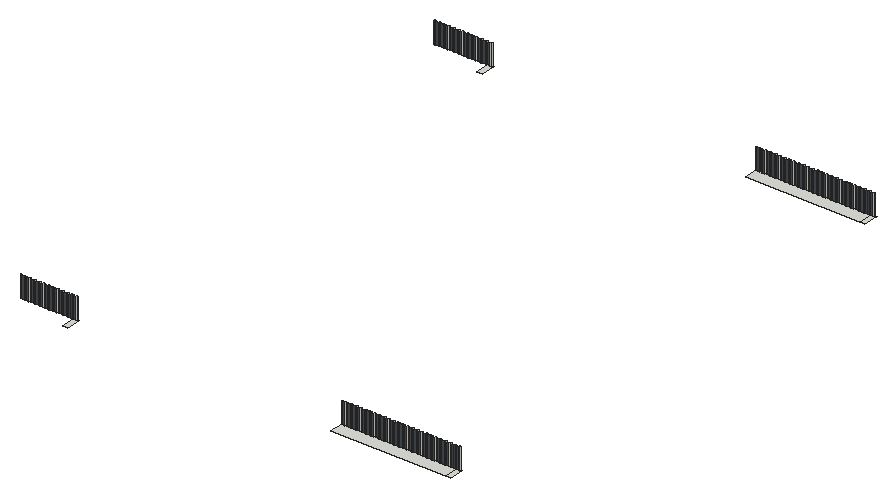
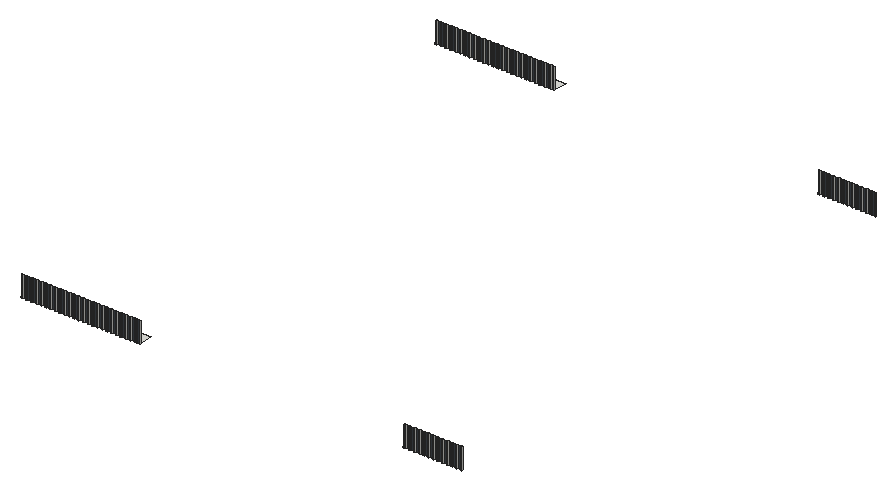
# SketchUp Ruby script. Lengths in inches.
U = 1.inch
M = Sketchup.active_model
def pt(a) = Geom::Point3d.new(a.map { |v| v * U })
def face(e, loops, mat)
  f = e.add_face(loops[0].map { |a| pt(a) })
  loops[1..].each { |l| e.add_face(l.map { |a| pt(a) }).erase! }
  f.material = f.back_material = mat if mat
  f
end
# faces: each face lists its corners as indices into pts; further lists are holes
def faces(e, pts, list, mat = nil) = list.each { |f| face(e, (f[0].is_a?(Array) ? f : [f]).map { |l| l.map { |i| pts[i] } }, mat) }
# xy, xz, yz: faces in a plane at the given z, y or x. An outline is a flat list of corners, or four numbers for a rectangle; further outlines are holes
def ring(l) = l.size == 4 ? [[l[0], l[1]], [l[2], l[1]], [l[2], l[3]], [l[0], l[3]]] : l.each_slice(2).to_a
def flat(e, list, mat, &to3) = list.each { |f| face(e, (f[0].is_a?(Array) ? f : [f]).map { |l| ring(l).map { |u, v| to3.(u, v) } }, mat) }
def xy(e, z, list, mat = nil) = flat(e, list, mat) { |x, y| [x, y, z] }
def xz(e, y, list, mat = nil) = flat(e, list, mat) { |x, z| [x, y, z] }
def yz(e, x, list, mat = nil) = flat(e, list, mat) { |y, z| [x, y, z] }
def lines(e, pts, list) = list.each { |a, b| e.add_line(pt(pts[a]), pt(pts[b])) }
# prism: a flat outline (further loops are holes) pulled along v
def prism(e, loops, v, mat = nil)
  f = face(e, loops, mat); d = Geom::Vector3d.new(v.map { |x| x * U })
  f.pushpull(f.normal.samedirection?(d) ? d.length : -d.length)
end
def box(e, o, s, mat = nil) = prism(e, [[o, [o[0] + s[0], o[1], o[2]], [o[0] + s[0], o[1] + s[1], o[2]], [o[0], o[1] + s[1], o[2]]]], [0, 0, s[2]], mat)
def at(x, y, z, deg = 0) = Geom::Transformation.translation(pt([x, y, z])) * Geom::Transformation.rotation(ORIGIN, Z_AXIS, deg.degrees)
def axes(o, x, y, z) = Geom::Transformation.new([*x, 0, *y, 0, *z, 0, *pt(o).to_a, 1])
def part(name) = M.definitions.add(name)
# library, detail: a bought-in or finely detailed component or shape, given as its bounding box
def library(name, o, s) = part(name).tap { |d| box(d.entities, o, s) }
def detail(e, o, s) = box(e.add_group.entities, o, s)
def put(e, d, t, mat = nil) = e.add_instance(d, t).tap { |i| i.material = mat if mat }
def group(e, t, mat = nil) = e.add_group.tap { |g| g.transformation = t; g.material = mat if mat }.entities
root = M.entities
M.materials.add("[Formica Blue]").color = [73, 80, 86]
xy(root,693.65,[[1078.41,412.04,1088.17,412.04,1088.17,437.1,1085.74,437.1,1085.74,438.72,1083.18,438.72,1083.18,437.1,1078.41,437.1],[1586.375,412.04,1802.84,412.04,1802.84,437.1,1801.29,437.1,1801.29,438.72,1798.73,438.72,1798.73,437.1,1792.39,437.1,1792.39,438.72,1789.84,438.72,1789.84,437.1,1783.5,437.1,1783.5,438.72,1780.95,438.72,1780.95,437.1,1774.61,437.1,1774.61,438.72,1772.05,438.72,1772.05,437.1,1765.72,437.1,1765.72,438.72,1763.16,438.72,1763.16,437.1,1756.83,437.1,1756.83,438.72,1754.27,438.72,1754.27,437.1,1747.9375,437.1,1747.9375,438.72,1745.38,438.72,1745.38,437.1,1739.05,437.1,1739.05,438.72,1736.49,438.72,1736.49,437.1,1730.16,437.1,1730.16,438.72,1727.6,438.72,1727.6,437.1,1721.26,437.1,1721.26,438.72,1718.71,438.72,1718.71,437.1,1712.375,437.1,1712.375,438.72,1709.82,438.72,1709.82,437.1,1703.48,437.1,1703.48,438.72,1700.92,438.72,1700.92,437.1,1694.59,437.1,1694.59,438.72,1692.03,438.72,1692.03,437.1,1685.7,437.1,1685.7,438.72,1683.14,438.72,1683.14,437.1,1676.81,437.1,1676.81,438.72,1674.25,438.72,1674.25,437.1,1667.92,437.1,1667.92,438.72,1665.36,438.72,1665.36,437.1,1659.03,437.1,1659.03,438.72,1656.47,438.72,1656.47,437.1,1650.13,437.1,1650.13,438.72,1647.58,438.72,1647.58,437.1,1641.24,437.1,1641.24,438.72,1638.69,438.72,1638.69,437.1,1632.35,437.1,1632.35,438.72,1629.79,438.72,1629.79,437.1,1623.46,437.1,1623.46,438.72,1620.9,438.72,1620.9,437.1,1614.57,437.1,1614.57,438.72,1612.01,438.72,1612.01,437.1,1605.68,437.1,1605.68,438.72,1603.12,438.72,1603.12,437.1,1596.79,437.1,1596.79,438.72,1592.81,438.72,1592.81,437.1,1586.47,437.1,1586.47,438.72,1586.375,438.72],[1802.84,412.04,1812.6,412.04,1812.6,437.1,1810.18,437.1,1810.18,438.72,1807.62,438.72,1807.62,437.1,1802.84,437.1],[1085.74,437.1,1088.17,438.72],[1810.18,437.1,1812.6,438.72],
  [1078.41,1392.39,1088.17,1392.39,1088.17,1417.45,1085.74,1417.45,1085.74,1419.07,1083.18,1419.07,1083.18,1417.45,1078.41,1417.45],[1586.375,1392.39,1802.84,1392.39,1802.84,1417.45,1801.29,1417.45,1801.29,1419.07,1798.73,1419.07,1798.73,1417.45,1792.39,1417.45,1792.39,1419.07,1789.84,1419.07,1789.84,1417.45,1783.5,1417.45,1783.5,1419.07,1780.95,1419.07,1780.95,1417.45,1774.61,1417.45,1774.61,1419.07,1772.05,1419.07,1772.05,1417.45,1765.72,1417.45,1765.72,1419.07,1763.16,1419.07,1763.16,1417.45,1756.83,1417.45,1756.83,1419.07,1754.27,1419.07,1754.27,1417.45,1747.9375,1417.45,1747.9375,1419.07,1745.38,1419.07,1745.38,1417.45,1739.05,1417.45,1739.05,1419.07,1736.49,1419.07,1736.49,1417.45,1730.16,1417.45,1730.16,1419.07,1727.6,1419.07,1727.6,1417.45,1721.26,1417.45,1721.26,1419.07,1718.71,1419.07,1718.71,1417.45,1712.375,1417.45,1712.375,1419.07,1709.82,1419.07,1709.82,1417.45,1703.48,1417.45,1703.48,1419.07,1700.92,1419.07,1700.92,1417.45,1694.59,1417.45,1694.59,1419.07,1692.03,1419.07,1692.03,1417.45,1685.7,1417.45,1685.7,1419.07,1683.14,1419.07,1683.14,1417.45,1676.81,1417.45,1676.81,1419.07,1674.25,1419.07,1674.25,1417.45,1667.92,1417.45,1667.92,1419.07,1665.36,1419.07,1665.36,1417.45,1659.03,1417.45,1659.03,1419.07,1656.47,1419.07,1656.47,1417.45,1650.13,1417.45,1650.13,1419.07,1647.58,1419.07,1647.58,1417.45,1641.24,1417.45,1641.24,1419.07,1638.69,1419.07,1638.69,1417.45,1632.35,1417.45,1632.35,1419.07,1629.79,1419.07,1629.79,1417.45,1623.46,1417.45,1623.46,1419.07,1620.9,1419.07,1620.9,1417.45,1614.57,1417.45,1614.57,1419.07,1612.01,1419.07,1612.01,1417.45,1605.68,1417.45,1605.68,1419.07,1603.12,1419.07,1603.12,1417.45,1596.79,1417.45,1596.79,1419.07,1592.81,1419.07,1592.81,1417.45,1586.47,1417.45,1586.47,1419.07,1586.375,1419.07],[1802.84,1392.39,1812.6,1392.39,1812.6,1417.45,1810.18,1417.45,1810.18,1419.07,1807.62,1419.07,1807.62,1417.45,1802.84,1417.45],[1085.74,1417.45,1088.17,1419.07],[1810.18,1417.45,1812.6,1419.07]])
xz(root,437.1,[[979.04,693.65,985.38,733.125],[987.9375,693.65,994.27,733.125],[996.83,693.65,1003.16,733.125],[1005.72,693.65,1012.05,733.125],[1014.61,693.65,1020.94,733.125],
  [1023.5,693.65,1029.83,733.125],[1032.39,693.65,1038.73,733.125],[1041.28,693.65,1047.62,733.125],[1050.17,693.65,1056.51,733.125],[1059.07,693.65,1065.4,733.125],
  [1067.96,693.65,1074.29,733.125],[1076.85,693.65,1083.18,733.125],[1586.47,693.65,1592.81,733.125],[1596.79,693.65,1603.12,733.125],[1605.68,693.65,1612.01,733.125],
  [1614.57,693.65,1620.9,733.125],[1623.46,693.65,1629.79,733.125],[1632.35,693.65,1638.69,733.125],[1641.24,693.65,1647.58,733.125],[1650.13,693.65,1656.47,733.125],
  [1659.03,693.65,1665.36,733.125],[1667.92,693.65,1674.25,733.125],[1676.81,693.65,1683.14,733.125],[1685.7,693.65,1692.03,733.125],[1694.59,693.65,1700.92,733.125],
  [1703.48,693.65,1709.82,733.125],[1712.375,693.65,1718.71,733.125],[1721.26,693.65,1727.6,733.125],[1730.16,693.65,1736.49,733.125],[1739.05,693.65,1745.38,733.125],
  [1747.9375,693.65,1754.27,733.125],[1756.83,693.65,1763.16,733.125],[1765.72,693.65,1772.05,733.125],[1774.61,693.65,1780.95,733.125],[1783.5,693.65,1789.84,733.125],
  [1792.39,693.65,1798.73,733.125],[1801.29,693.65,1807.62,733.125]],"[Formica Blue]")
xz(root,438.72,[[1586.375,693.65,1586.47,733.125]])
xz(root,438.72,[[976.49,693.65,979.04,733.125],[985.38,693.65,987.9375,733.125],[994.27,693.65,996.83,733.125],[1003.16,693.65,1005.72,733.125],[1012.05,693.65,1014.61,733.125],
  [1020.94,693.65,1023.5,733.125],[1029.83,693.65,1032.39,733.125],[1038.73,693.65,1041.28,733.125],[1047.62,693.65,1050.17,733.125],[1056.51,693.65,1059.07,733.125],
  [1065.4,693.65,1067.96,733.125],[1074.29,693.65,1076.85,733.125],[1083.18,693.65,1085.74,733.125],[1592.81,693.65,1596.79,733.125],[1603.12,693.65,1605.68,733.125],
  [1612.01,693.65,1614.57,733.125],[1620.9,693.65,1623.46,733.125],[1629.79,693.65,1632.35,733.125],[1638.69,693.65,1641.24,733.125],[1647.58,693.65,1650.13,733.125],
  [1656.47,693.65,1659.03,733.125],[1665.36,693.65,1667.92,733.125],[1674.25,693.65,1676.81,733.125],[1683.14,693.65,1685.7,733.125],[1692.03,693.65,1694.59,733.125],
  [1700.92,693.65,1703.48,733.125],[1709.82,693.65,1712.375,733.125],[1718.71,693.65,1721.26,733.125],[1727.6,693.65,1730.16,733.125],[1736.49,693.65,1739.05,733.125],
  [1745.38,693.65,1747.9375,733.125],[1754.27,693.65,1756.83,733.125],[1763.16,693.65,1765.72,733.125],[1772.05,693.65,1774.61,733.125],[1780.95,693.65,1783.5,733.125],
  [1789.84,693.65,1792.39,733.125],[1798.73,693.65,1801.29,733.125],[1807.62,693.65,1810.18,733.125]],"[Formica Blue]")
xz(root,1417.45,[[979.04,693.65,985.38,733.125],[987.9375,693.65,994.27,733.125],[996.83,693.65,1003.16,733.125],[1005.72,693.65,1012.05,733.125],[1014.61,693.65,1020.94,733.125],
  [1023.5,693.65,1029.83,733.125],[1032.39,693.65,1038.73,733.125],[1041.28,693.65,1047.62,733.125],[1050.17,693.65,1056.51,733.125],[1059.07,693.65,1065.4,733.125],
  [1067.96,693.65,1074.29,733.125],[1076.85,693.65,1083.18,733.125],[1586.47,693.65,1592.81,733.125],[1596.79,693.65,1603.12,733.125],[1605.68,693.65,1612.01,733.125],
  [1614.57,693.65,1620.9,733.125],[1623.46,693.65,1629.79,733.125],[1632.35,693.65,1638.69,733.125],[1641.24,693.65,1647.58,733.125],[1650.13,693.65,1656.47,733.125],
  [1659.03,693.65,1665.36,733.125],[1667.92,693.65,1674.25,733.125],[1676.81,693.65,1683.14,733.125],[1685.7,693.65,1692.03,733.125],[1694.59,693.65,1700.92,733.125],
  [1703.48,693.65,1709.82,733.125],[1712.375,693.65,1718.71,733.125],[1721.26,693.65,1727.6,733.125],[1730.16,693.65,1736.49,733.125],[1739.05,693.65,1745.38,733.125],
  [1747.9375,693.65,1754.27,733.125],[1756.83,693.65,1763.16,733.125],[1765.72,693.65,1772.05,733.125],[1774.61,693.65,1780.95,733.125],[1783.5,693.65,1789.84,733.125],
  [1792.39,693.65,1798.73,733.125],[1801.29,693.65,1807.62,733.125]],"[Formica Blue]")
xz(root,1419.07,[[1586.375,693.65,1586.47,733.125]])
xz(root,1419.07,[[976.49,693.65,979.04,733.125],[985.38,693.65,987.9375,733.125],[994.27,693.65,996.83,733.125],[1003.16,693.65,1005.72,733.125],[1012.05,693.65,1014.61,733.125],
  [1020.94,693.65,1023.5,733.125],[1029.83,693.65,1032.39,733.125],[1038.73,693.65,1041.28,733.125],[1047.62,693.65,1050.17,733.125],[1056.51,693.65,1059.07,733.125],
  [1065.4,693.65,1067.96,733.125],[1074.29,693.65,1076.85,733.125],[1083.18,693.65,1085.74,733.125],[1592.81,693.65,1596.79,733.125],[1603.12,693.65,1605.68,733.125],
  [1612.01,693.65,1614.57,733.125],[1620.9,693.65,1623.46,733.125],[1629.79,693.65,1632.35,733.125],[1638.69,693.65,1641.24,733.125],[1647.58,693.65,1650.13,733.125],
  [1656.47,693.65,1659.03,733.125],[1665.36,693.65,1667.92,733.125],[1674.25,693.65,1676.81,733.125],[1683.14,693.65,1685.7,733.125],[1692.03,693.65,1694.59,733.125],
  [1700.92,693.65,1703.48,733.125],[1709.82,693.65,1712.375,733.125],[1718.71,693.65,1721.26,733.125],[1727.6,693.65,1730.16,733.125],[1736.49,693.65,1739.05,733.125],
  [1745.38,693.65,1747.9375,733.125],[1754.27,693.65,1756.83,733.125],[1763.16,693.65,1765.72,733.125],[1772.05,693.65,1774.61,733.125],[1780.95,693.65,1783.5,733.125],
  [1789.84,693.65,1792.39,733.125],[1798.73,693.65,1801.29,733.125],[1807.62,693.65,1810.18,733.125]],"[Formica Blue]")
yz(root,976.49,[[1417.45,693.65,1419.07,733.125]])
yz(root,979.04,[[437.1,693.65,438.72,733.125],[1417.45,693.65,1419.07,733.125]])
yz(root,985.38,[[437.1,693.65,438.72,733.125],[1417.45,693.65,1419.07,733.125]])
yz(root,987.9375,[[437.1,693.65,438.72,733.125],[1417.45,693.65,1419.07,733.125]])
yz(root,994.27,[[437.1,693.65,438.72,733.125],[1417.45,693.65,1419.07,733.125]])
yz(root,996.83,[[437.1,693.65,438.72,733.125],[1417.45,693.65,1419.07,733.125]])
yz(root,1003.16,[[437.1,693.65,438.72,733.125],[1417.45,693.65,1419.07,733.125]])
yz(root,1005.72,[[437.1,693.65,438.72,733.125],[1417.45,693.65,1419.07,733.125]])
yz(root,1012.05,[[437.1,693.65,438.72,733.125],[1417.45,693.65,1419.07,733.125]])
yz(root,1014.61,[[437.1,693.65,438.72,733.125],[1417.45,693.65,1419.07,733.125]])
yz(root,1020.94,[[437.1,693.65,438.72,733.125],[1417.45,693.65,1419.07,733.125]])
yz(root,1023.5,[[437.1,693.65,438.72,733.125],[1417.45,693.65,1419.07,733.125]])
yz(root,1029.83,[[437.1,693.65,438.72,733.125],[1417.45,693.65,1419.07,733.125]])
yz(root,1032.39,[[437.1,693.65,438.72,733.125],[1417.45,693.65,1419.07,733.125]])
yz(root,1038.73,[[437.1,693.65,438.72,733.125],[1417.45,693.65,1419.07,733.125]])
yz(root,1041.28,[[437.1,693.65,438.72,733.125],[1417.45,693.65,1419.07,733.125]])
yz(root,1047.62,[[437.1,693.65,438.72,733.125],[1417.45,693.65,1419.07,733.125]])
yz(root,1050.17,[[437.1,693.65,438.72,733.125],[1417.45,693.65,1419.07,733.125]])
yz(root,1056.51,[[437.1,693.65,438.72,733.125],[1417.45,693.65,1419.07,733.125]])
yz(root,1059.07,[[437.1,693.65,438.72,733.125],[1417.45,693.65,1419.07,733.125]])
yz(root,1065.4,[[437.1,693.65,438.72,733.125],[1417.45,693.65,1419.07,733.125]])
yz(root,1067.96,[[437.1,693.65,438.72,733.125],[1417.45,693.65,1419.07,733.125]])
yz(root,1074.29,[[437.1,693.65,438.72,733.125],[1417.45,693.65,1419.07,733.125]],"[Formica Blue]")
yz(root,1076.85,[[437.1,693.65,438.72,733.125],[1417.45,693.65,1419.07,733.125]])
yz(root,1083.18,[[437.1,693.65,438.72,733.125],[1417.45,693.65,1419.07,733.125]])
yz(root,1085.74,[[437.1,693.65,438.72,733.125],[1417.45,693.65,1419.07,733.125]])
yz(root,1586.47,[[437.1,693.65,438.72,733.125],[1417.45,693.65,1419.07,733.125]])
yz(root,1592.81,[[437.1,693.65,438.72,733.125],[1417.45,693.65,1419.07,733.125]])
yz(root,1596.79,[[437.1,693.65,438.72,733.125],[1417.45,693.65,1419.07,733.125]])
yz(root,1603.12,[[437.1,693.65,438.72,733.125],[1417.45,693.65,1419.07,733.125]])
yz(root,1605.68,[[437.1,693.65,438.72,733.125],[1417.45,693.65,1419.07,733.125]])
yz(root,1612.01,[[437.1,693.65,438.72,733.125],[1417.45,693.65,1419.07,733.125]])
yz(root,1614.57,[[437.1,693.65,438.72,733.125],[1417.45,693.65,1419.07,733.125]])
yz(root,1620.9,[[437.1,693.65,438.72,733.125],[1417.45,693.65,1419.07,733.125]])
yz(root,1623.46,[[437.1,693.65,438.72,733.125],[1417.45,693.65,1419.07,733.125]])
yz(root,1629.79,[[437.1,693.65,438.72,733.125],[1417.45,693.65,1419.07,733.125]])
yz(root,1632.35,[[437.1,693.65,438.72,733.125],[1417.45,693.65,1419.07,733.125]])
yz(root,1638.69,[[437.1,693.65,438.72,733.125],[1417.45,693.65,1419.07,733.125]])
yz(root,1641.24,[[437.1,693.65,438.72,733.125],[1417.45,693.65,1419.07,733.125]])
yz(root,1647.58,[[437.1,693.65,438.72,733.125],[1417.45,693.65,1419.07,733.125]])
yz(root,1650.13,[[437.1,693.65,438.72,733.125],[1417.45,693.65,1419.07,733.125]])
yz(root,1656.47,[[437.1,693.65,438.72,733.125],[1417.45,693.65,1419.07,733.125]])
yz(root,1659.03,[[437.1,693.65,438.72,733.125],[1417.45,693.65,1419.07,733.125]])
yz(root,1665.36,[[437.1,693.65,438.72,733.125],[1417.45,693.65,1419.07,733.125]])
yz(root,1667.92,[[437.1,693.65,438.72,733.125],[1417.45,693.65,1419.07,733.125]])
yz(root,1674.25,[[437.1,693.65,438.72,733.125],[1417.45,693.65,1419.07,733.125]])
yz(root,1676.81,[[437.1,693.65,438.72,733.125],[1417.45,693.65,1419.07,733.125]])
yz(root,1683.14,[[437.1,693.65,438.72,733.125],[1417.45,693.65,1419.07,733.125]])
yz(root,1685.7,[[437.1,693.65,438.72,733.125],[1417.45,693.65,1419.07,733.125]])
yz(root,1692.03,[[437.1,693.65,438.72,733.125],[1417.45,693.65,1419.07,733.125]])
yz(root,1694.59,[[437.1,693.65,438.72,733.125],[1417.45,693.65,1419.07,733.125]])
yz(root,1700.92,[[437.1,693.65,438.72,733.125],[1417.45,693.65,1419.07,733.125]])
yz(root,1703.48,[[437.1,693.65,438.72,733.125],[1417.45,693.65,1419.07,733.125]])
yz(root,1709.82,[[437.1,693.65,438.72,733.125],[1417.45,693.65,1419.07,733.125]])
yz(root,1712.375,[[437.1,693.65,438.72,733.125],[1417.45,693.65,1419.07,733.125]])
yz(root,1718.71,[[437.1,693.65,438.72,733.125],[1417.45,693.65,1419.07,733.125]])
yz(root,1721.26,[[437.1,693.65,438.72,733.125],[1417.45,693.65,1419.07,733.125]])
yz(root,1727.6,[[437.1,693.65,438.72,733.125],[1417.45,693.65,1419.07,733.125]])
yz(root,1730.16,[[437.1,693.65,438.72,733.125],[1417.45,693.65,1419.07,733.125]])
yz(root,1736.49,[[437.1,693.65,438.72,733.125],[1417.45,693.65,1419.07,733.125]])
yz(root,1739.05,[[437.1,693.65,438.72,733.125],[1417.45,693.65,1419.07,733.125]])
yz(root,1745.38,[[437.1,693.65,438.72,733.125],[1417.45,693.65,1419.07,733.125]])
yz(root,1747.9375,[[437.1,693.65,438.72,733.125],[1417.45,693.65,1419.07,733.125]])
yz(root,1754.27,[[437.1,693.65,438.72,733.125],[1417.45,693.65,1419.07,733.125]])
yz(root,1756.83,[[437.1,693.65,438.72,733.125],[1417.45,693.65,1419.07,733.125]])
yz(root,1763.16,[[437.1,693.65,438.72,733.125],[1417.45,693.65,1419.07,733.125]])
yz(root,1765.72,[[437.1,693.65,438.72,733.125],[1417.45,693.65,1419.07,733.125]])
yz(root,1772.05,[[437.1,693.65,438.72,733.125],[1417.45,693.65,1419.07,733.125]])
yz(root,1774.61,[[437.1,693.65,438.72,733.125],[1417.45,693.65,1419.07,733.125]])
yz(root,1780.95,[[437.1,693.65,438.72,733.125],[1417.45,693.65,1419.07,733.125]])
yz(root,1783.5,[[437.1,693.65,438.72,733.125],[1417.45,693.65,1419.07,733.125]])
yz(root,1789.84,[[437.1,693.65,438.72,733.125],[1417.45,693.65,1419.07,733.125]])
yz(root,1792.39,[[437.1,693.65,438.72,733.125],[1417.45,693.65,1419.07,733.125]])
yz(root,1798.73,[[437.1,693.65,438.72,733.125],[1417.45,693.65,1419.07,733.125]],"[Formica Blue]")
yz(root,1801.29,[[437.1,693.65,438.72,733.125],[1417.45,693.65,1419.07,733.125]])
yz(root,1807.62,[[437.1,693.65,438.72,733.125],[1417.45,693.65,1419.07,733.125]])
yz(root,1810.18,[[437.1,693.65,438.72,733.125],[1417.45,693.65,1419.07,733.125]])
